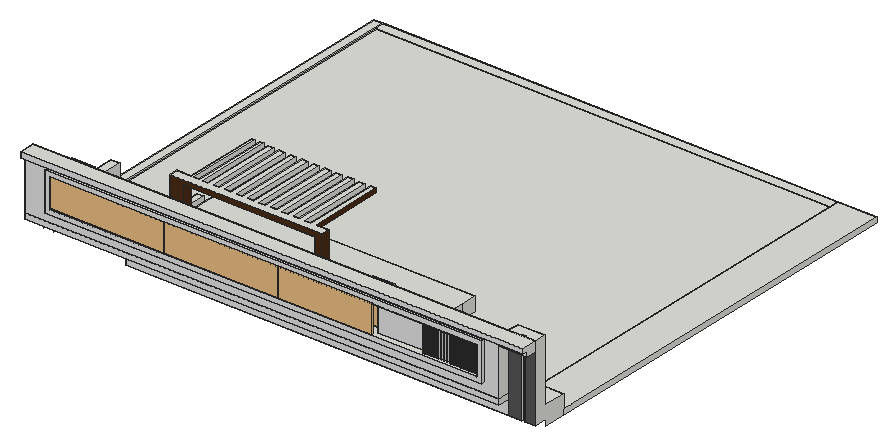
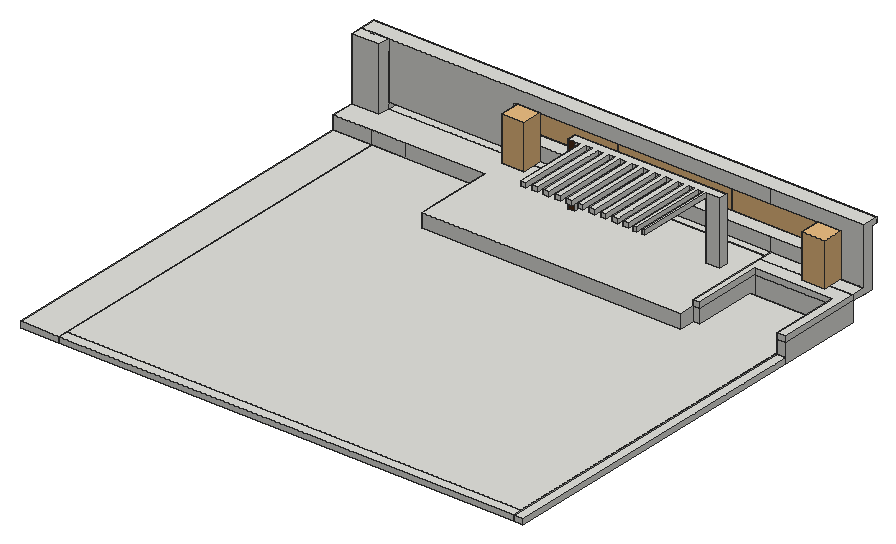
# SketchUp Ruby script. Lengths in inches.
U = 1.inch
M = Sketchup.active_model
def pt(a) = Geom::Point3d.new(a.map { |v| v * U })
def face(e, loops, mat)
  f = e.add_face(loops[0].map { |a| pt(a) })
  loops[1..].each { |l| e.add_face(l.map { |a| pt(a) }).erase! }
  f.material = f.back_material = mat if mat
  f
end
# faces: each face lists its corners as indices into pts; further lists are holes
def faces(e, pts, list, mat = nil) = list.each { |f| face(e, (f[0].is_a?(Array) ? f : [f]).map { |l| l.map { |i| pts[i] } }, mat) }
# xy, xz, yz: faces in a plane at the given z, y or x. An outline is a flat list of corners, or four numbers for a rectangle; further outlines are holes
def ring(l) = l.size == 4 ? [[l[0], l[1]], [l[2], l[1]], [l[2], l[3]], [l[0], l[3]]] : l.each_slice(2).to_a
def flat(e, list, mat, &to3) = list.each { |f| face(e, (f[0].is_a?(Array) ? f : [f]).map { |l| ring(l).map { |u, v| to3.(u, v) } }, mat) }
def xy(e, z, list, mat = nil) = flat(e, list, mat) { |x, y| [x, y, z] }
def xz(e, y, list, mat = nil) = flat(e, list, mat) { |x, z| [x, y, z] }
def yz(e, x, list, mat = nil) = flat(e, list, mat) { |y, z| [x, y, z] }
def lines(e, pts, list) = list.each { |a, b| e.add_line(pt(pts[a]), pt(pts[b])) }
# prism: a flat outline (further loops are holes) pulled along v
def prism(e, loops, v, mat = nil)
  f = face(e, loops, mat); d = Geom::Vector3d.new(v.map { |x| x * U })
  f.pushpull(f.normal.samedirection?(d) ? d.length : -d.length)
end
def box(e, o, s, mat = nil) = prism(e, [[o, [o[0] + s[0], o[1], o[2]], [o[0] + s[0], o[1] + s[1], o[2]], [o[0], o[1] + s[1], o[2]]]], [0, 0, s[2]], mat)
def at(x, y, z, deg = 0) = Geom::Transformation.translation(pt([x, y, z])) * Geom::Transformation.rotation(ORIGIN, Z_AXIS, deg.degrees)
def axes(o, x, y, z) = Geom::Transformation.new([*x, 0, *y, 0, *z, 0, *pt(o).to_a, 1])
def part(name) = M.definitions.add(name)
# library, detail: a bought-in or finely detailed component or shape, given as its bounding box
def library(name, o, s) = part(name).tap { |d| box(d.entities, o, s) }
def detail(e, o, s) = box(e.add_group.entities, o, s)
def put(e, d, t, mat = nil) = e.add_instance(d, t).tap { |i| i.material = mat if mat }
def group(e, t, mat = nil) = e.add_group.tap { |g| g.transformation = t; g.material = mat if mat }.entities
root = M.entities
M.materials.add("[Color M01]").color = [226, 226, 226]
M.materials.add("[Color M06]").color = [86, 86, 86]
M.materials.add("[Wood Veneer 01]").color = [76, 44, 23]
c1 = library("SPOT",[0,0,1.68],[5.4375,5.4375,6.28])
c2 = library("Yukka",[-2.74,-1.93,0],[38.67,34.64,74.8125])
c3 = part("glass-railing")
detail(c3.entities,[0,0,0],[1.26,75.59,33.1875])
xy(root,510,[[303.12,279.2,303.12,683.75,784.56,683.75,784.56,279.2,665.11,279.2,665.11,362.65,390.34,362.65,390.34,345.71,383.72,345.71,383.72,279.2],[383.72,279.2,390.34,345.71],[390.34,279.2,665.11,362.65],[784.56,279.2,825.43,694.43],[292.06,345.71,301.28,694.43],
  [301.28,683.75,784.56,694.43]])
xy(root,515.875,[[657.09,242.18,657.09,263.24,751.93,263.24,751.93,256.61,754.62,256.61,754.62,263.24,761.98,263.24,761.98,256.61,784.56,256.61,784.56,242.18],[784.56,242.18,784.56,256.61,811.07,256.61,811.07,258.49,814.72,258.49,814.72,256.61,825.43,256.61,825.43,242.18,813.93,242.18,813.93,244.11,810.6,244.11,810.6,242.18]])
xy(root,515.875,[[[390.34,242.18,657.09,345.71],[511.65,248.63,512.53,248.63,512.53,249.32,515.36,249.32,515.36,250.63,516,250.63,516,249.32,518.83,249.32,518.83,250.63,519.47,250.63,519.47,249.32,522.3,249.32,522.3,250.63,522.9375,250.63,522.9375,249.32,525.77,249.32,525.77,250.63,526.41,250.63,526.41,249.32,529.24,249.32,529.24,250.63,529.78,250.63,529.78,248.63,530.65,248.63,530.65,269.63,511.65,269.63],[595.53,289.875,596.83,289.96,598.07,290.37,599.16,291.09,600.02,292.07,600.61,293.24,600.87,294.52,600.79,295.82,600.37,297.06,599.65,298.14,598.67,299.01,597.51,299.59,596.23,299.85,594.92,299.77,593.6875,299.36,592.6,298.64,591.73,297.66,591.15,296.49,590.89,295.21,590.97,293.91,591.39,292.67,592.11,291.58,593.08,290.72,594.25,290.14],[447.91,289.875,449.21,289.96,450.45,290.37,451.53,291.09,452.4,292.07,452.98,293.24,453.24,294.52,453.16,295.82,452.75,297.06,452.03,298.14,451.05,299.01,449.88,299.59,448.6,299.85,447.3,299.77,446.0625,299.36,444.97,298.64,444.11,297.66,443.53,296.49,443.27,295.21,443.35,293.91,443.76,292.67,444.48,291.58,445.46,290.72,446.625,290.14]]],"[Wood Veneer 01]")
xy(root,516,[[303.12,279.2,784.56,683.75],[784.56,279.2,825.43,694.43],[292.06,345.71,301.28,694.43],[301.28,683.75,784.56,694.43]])
xy(root,516.9375,[[595.53,289.875,594.25,290.14,593.08,290.72,592.11,291.58,591.39,292.67,590.97,293.91,590.89,295.21,591.15,296.49,591.73,297.66,592.6,298.64,593.6875,299.36,594.92,299.77,596.23,299.85,597.51,299.59,598.67,299.01,599.65,298.14,600.37,297.06,600.79,295.82,600.87,294.52,600.61,293.24,600.02,292.07,599.16,291.09,598.07,290.37,596.83,289.96]])
xy(root,517.375,[[447.91,289.875,446.625,290.14,445.46,290.72,444.48,291.58,443.76,292.67,443.35,293.91,443.27,295.21,443.53,296.49,444.11,297.66,444.97,298.64,446.0625,299.36,447.3,299.77,448.6,299.85,449.88,299.59,451.05,299.01,452.03,298.14,452.75,297.06,453.16,295.82,453.24,294.52,452.98,293.24,452.4,292.07,451.53,291.09,450.45,290.37,449.21,289.96]])
xy(root,519.6875,[[302.78,256.61,380.53,263.24]])
xy(root,530.25,[[292.06,231.11,390.34,242.18],[390.34,231.11,795.77,242.18],[[390.34,242.18,795.77,242.18,797.0625,254.92,825.43,254.92,825.43,279.2,665.11,279.2,665.11,362.65,390.34,362.65],[413.19,272.63,428.05,281.82],[567.24,272.63,573.99,281.82]]])
xy(root,536.3125,[[292.06,231.11,795.77,242.18],[292.06,242.18,390.34,256.61],[292.06,256.61,390.34,256.61,390.34,345.71,383.72,345.71,383.72,272.46,301.28,272.46,301.28,345.71,292.06,345.71]])
xy(root,546.15,[[316.49,227.68,779.86,231.11]])
xy(root,550.91,[[321.25,227.68,775.1,227.68,775.1,232.24,773.26,232.24,773.26,234.93,771.98,234.93,771.98,232.24,770.13,232.24,770.13,234.93,768.85,234.93,768.85,232.24,767.01,232.24,767.01,234.93,765.73,234.93,765.73,232.24,763.88,232.24,763.88,234.93,762.6,234.93,762.6,232.24,760.76,232.24,760.76,234.93,759.48,234.93,759.48,232.24,757.63,232.24,757.63,234.93,756.35,234.93,756.35,232.24,754.51,232.24,754.51,234.93,753.23,234.93,753.23,232.24,751.38,232.24,751.38,234.93,750.1,234.93,750.1,232.24,748.26,232.24,748.26,234.93,746.98,234.93,746.98,232.24,745.13,232.24,745.13,234.93,743.85,234.93,743.85,232.24,742.01,232.24,742.01,234.93,740.73,234.93,740.73,232.24,738.88,232.24,738.88,234.93,737.6,234.93,737.6,232.24,735.76,232.24,735.76,234.93,734.48,234.93,734.48,232.24,732.63,232.24,732.63,234.93,731.35,234.93,731.35,232.24,729.51,232.24,729.51,234.93,728.23,234.93,728.23,232.24,726.38,232.24,726.38,234.93,725.1,234.93,725.1,232.24,723.26,232.24,723.26,234.93,721.98,234.93,721.98,232.24,720.13,232.24,720.13,234.93,719.1,234.93,719.1,232.24,717.26,232.24,717.26,234.93,716.23,234.93,716.23,231.3,714.38,231.3,714.38,234.93,663.67,234.93,663.67,242.18,321.25,242.18],[714.38,231.3,716.23,233.99],[717.26,232.24,719.1,234.93],[720.13,232.24,721.98,234.93],[723.26,232.24,725.1,234.93],
  [726.38,232.24,728.23,234.93],[729.51,232.24,731.35,234.93],[732.63,232.24,734.48,234.93],[735.76,232.24,737.6,234.93],[738.88,232.24,740.73,234.93],
  [742.01,232.24,743.85,234.93],[745.13,232.24,746.98,234.93],[748.26,232.24,750.1,234.93],[751.38,232.24,753.23,234.93],[754.51,232.24,756.35,234.93],
  [757.63,232.24,759.48,234.93],[760.76,232.24,762.6,234.93],[763.88,232.24,765.73,234.93],[767.01,232.24,768.85,234.93],[770.13,232.24,771.98,234.18],
  [773.26,232.24,775.1,232.99],[773.26,232.99,775.1,234.93],[714.38,233.99,716.23,234.3],[770.13,234.18,771.98,234.61],[770.13,234.61,771.98,234.93]])
xy(root,582.02,[[321.25,227.68,321.25,242.18,663.67,242.18,663.67,234.93,714.38,234.93,714.38,231.3,716.23,231.3,716.23,234.93,717.26,234.93,717.26,232.24,719.1,232.24,719.1,234.93,720.13,234.93,720.13,232.24,721.98,232.24,721.98,234.93,723.26,234.93,723.26,232.24,725.1,232.24,725.1,234.93,726.38,234.93,726.38,232.24,728.23,232.24,728.23,234.93,729.51,234.93,729.51,232.24,731.35,232.24,731.35,234.93,732.63,234.93,732.63,232.24,734.48,232.24,734.48,234.93,735.76,234.93,735.76,232.24,737.6,232.24,737.6,234.93,738.88,234.93,738.88,232.24,740.73,232.24,740.73,234.93,742.01,234.93,742.01,232.24,743.85,232.24,743.85,234.93,745.13,234.93,745.13,232.24,746.98,232.24,746.98,234.93,748.26,234.93,748.26,232.24,750.1,232.24,750.1,234.93,751.38,234.93,751.38,232.24,753.23,232.24,753.23,234.93,754.51,234.93,754.51,232.24,756.35,232.24,756.35,234.93,757.63,234.93,757.63,232.24,759.48,232.24,759.48,234.93,760.76,234.93,760.76,232.24,762.6,232.24,762.6,234.93,763.88,234.93,763.88,232.24,765.73,232.24,765.73,234.93,767.01,234.93,767.01,232.24,768.85,232.24,768.85,234.93,770.13,234.93,770.13,232.24,771.98,232.24,771.98,234.93,773.26,234.93,773.26,232.24,775.1,232.24,775.1,227.68],[714.38,231.3,716.23,233.99],[717.26,232.24,719.1,234.93],[720.13,232.24,721.98,234.93],[723.26,232.24,725.1,234.93],
  [726.38,232.24,728.23,234.93],[729.51,232.24,731.35,234.93],[732.63,232.24,734.48,234.93],[735.76,232.24,737.6,234.93],[738.88,232.24,740.73,234.93],
  [742.01,232.24,743.85,234.93],[745.13,232.24,746.98,234.93],[748.26,232.24,750.1,234.93],[751.38,232.24,753.23,234.93],[754.51,232.24,756.35,234.93],
  [757.63,232.24,759.48,234.93],[760.76,232.24,762.6,234.93],[763.88,232.24,765.73,234.93],[767.01,232.24,768.85,234.93],[770.13,232.24,771.98,234.18],
  [773.26,232.24,775.1,232.99],[773.26,232.99,775.1,234.93],[714.38,233.99,716.23,234.3],[770.13,234.18,771.98,234.61],[770.13,234.61,771.98,234.93]])
xy(root,586.3,[[795.77,231.11,825.43,242.18]])
xy(root,586.78,[[316.49,227.68,779.86,231.11]])
xy(root,591.86,[[428.05,272.63,428.05,362.65,431.14,362.65,431.14,281.82,436.78,281.82,436.78,362.65,440.71,362.65,440.71,281.82,445.99,281.82,445.99,361.33,452.05,361.33,452.05,281.82,458.11,281.82,458.11,361.33,464.18,361.33,464.18,281.82,470.24,281.82,470.24,361.33,476.3,361.33,476.3,281.82,482.36,281.82,482.36,361.33,488.43,361.33,488.43,281.82,494.49,281.82,494.49,361.33,500.55,361.33,500.55,281.82,506.61,281.82,506.61,361.33,512.68,361.33,512.68,281.82,518.74,281.82,518.74,361.33,524.8,361.33,524.8,281.82,530.86,281.82,530.86,361.33,536.93,361.33,536.93,281.82,542.99,281.82,542.99,361.33,549.05,361.33,549.05,281.82,555.11,281.82,555.11,361.33,561.18,361.33,561.18,281.82,567.24,281.82,567.24,272.63]],"[Wood Veneer 01]")
xy(root,596.625,[[292.06,225.49,825.43,242.18],[795.77,242.18,810.6,242.18,810.6,244.11,813.93,244.11,813.93,242.18,825.43,242.18,825.43,254.92,797.0625,254.92],[413.19,272.63,573.99,272.63,573.99,281.82,561.18,281.82,561.18,361.33,555.11,361.33,555.11,281.82,549.05,281.82,549.05,361.33,542.99,361.33,542.99,281.82,536.93,281.82,536.93,361.33,530.86,361.33,530.86,281.82,524.8,281.82,524.8,361.33,518.74,361.33,518.74,281.82,512.68,281.82,512.68,361.33,506.61,361.33,506.61,281.82,500.55,281.82,500.55,361.33,494.49,361.33,494.49,281.82,488.43,281.82,488.43,361.33,482.36,361.33,482.36,281.82,476.3,281.82,476.3,361.33,470.24,361.33,470.24,281.82,464.18,281.82,464.18,361.33,458.11,361.33,458.11,281.82,452.05,281.82,452.05,361.33,445.99,361.33,445.99,281.82,440.71,281.82,440.71,362.65,436.78,362.65,436.78,281.82,431.14,281.82,431.14,362.65,428.05,362.65,428.05,281.82,413.19,281.82]])
xz(root,225.49,[[292.06,590.76,825.43,591.46,825.43,596.625,292.06,596.625]],"[Color M01]")
xz(root,227.68,[[[316.49,546.15,779.86,586.78],[321.25,550.91,775.1,582.02]]],"[Color M01]")
xz(root,231.11,[[292.06,530.25,795.77,536.3125],[[292.06,536.3125,795.77,536.3125,795.77,586.3,825.43,586.3,825.43,591.46,292.06,590.76],[316.49,546.15,779.86,586.78]]],"[Color M01]")
xz(root,231.3,[[714.38,550.91,716.23,582.02]],"[Wood Veneer 01]")
xz(root,232.24,[[717.26,550.91,719.1,582.02],[720.13,550.91,721.98,582.02],[723.26,550.91,725.1,582.02],[726.38,550.91,728.23,582.02],[729.51,550.91,731.35,582.02],
  [732.63,550.91,734.48,582.02],[735.76,550.91,737.6,582.02],[738.88,550.91,740.73,582.02],[742.01,550.91,743.85,582.02],[745.13,550.91,746.98,582.02],
  [748.26,550.91,750.1,582.02],[751.38,550.91,753.23,582.02],[754.51,550.91,756.35,582.02],[757.63,550.91,759.48,582.02],[760.76,550.91,762.6,582.02],
  [763.88,550.91,765.73,582.02],[767.01,550.91,768.85,582.02],[770.13,550.91,771.98,582.02],[773.26,550.91,775.1,582.02]],"[Wood Veneer 01]")
xz(root,232.99,[[773.26,550.91,775.1,582.02]])
xz(root,233.99,[[714.38,550.91,716.23,582.02]])
xz(root,234.18,[[770.13,550.91,771.98,582.02]])
xz(root,234.3,[[714.38,550.91,716.23,582.02]])
xz(root,234.61,[[770.13,550.91,771.98,582.02]])
xz(root,234.93,[[716.23,550.91,717.26,582.02],[717.26,550.91,719.1,582.02],[719.1,550.91,720.13,582.02],[720.13,550.91,721.98,582.02],[721.98,550.91,723.26,582.02],
  [723.26,550.91,725.1,582.02],[725.1,550.91,726.38,582.02],[726.38,550.91,728.23,582.02],[728.23,550.91,729.51,582.02],[729.51,550.91,731.35,582.02],
  [731.35,550.91,732.63,582.02],[732.63,550.91,734.48,582.02],[734.48,550.91,735.76,582.02],[735.76,550.91,737.6,582.02],[737.6,550.91,738.88,582.02],
  [738.88,550.91,740.73,582.02],[740.73,550.91,742.01,582.02],[742.01,550.91,743.85,582.02],[743.85,550.91,745.13,582.02],[745.13,550.91,746.98,582.02],
  [746.98,550.91,748.26,582.02],[748.26,550.91,750.1,582.02],[750.1,550.91,751.38,582.02],[751.38,550.91,753.23,582.02],[753.23,550.91,754.51,582.02],
  [754.51,550.91,756.35,582.02],[756.35,550.91,757.63,582.02],[757.63,550.91,759.48,582.02],[759.48,550.91,760.76,582.02],[760.76,550.91,762.6,582.02],
  [762.6,550.91,763.88,582.02],[763.88,550.91,765.73,582.02],[765.73,550.91,767.01,582.02],[767.01,550.91,768.85,582.02],[768.85,550.91,770.13,582.02],
  [770.13,550.91,771.98,582.02],[771.98,550.91,773.26,582.02],[773.26,550.91,775.1,582.02]])
xz(root,234.93,[[663.67,550.91,714.38,582.02]],"[Color M01]")
xz(root,242.18,[[292.06,530.25,390.34,536.3125],[292.06,536.3125,292.06,596.625,390.34,596.625,390.34,582.02,321.25,582.02,321.25,550.91,390.34,550.91,390.34,536.3125],[390.34,536.3125,390.34,550.91,663.67,550.91,663.67,582.02,390.34,582.02,390.34,596.625,795.77,596.625,795.77,536.3125],[795.77,586.3,810.6,596.625],[810.6,586.3,813.93,596.625],
  [813.93,586.3,825.43,596.625]])
xz(root,242.18,[[390.34,515.875,795.77,530.25]],"[Color M01]")
xz(root,242.18,[[795.77,515.875,810.6,586.3],[813.93,515.875,825.43,586.3]],"[Color M06]")
xz(root,254.92,[[797.0625,530.25,825.43,596.625]])
xz(root,256.61,[[292.06,530.25,390.34,536.3125]])
xz(root,272.46,[[301.28,510,383.72,530.25],[301.28,530.25,383.72,536.3125]])
xz(root,272.63,[[413.19,530.25,428.05,530.25,428.05,591.86,567.24,591.86,567.24,530.25,573.99,530.25,573.99,596.625,413.19,596.625]],"[Wood Veneer 01]")
xz(root,279.2,[[303.12,510,665.11,516],[665.11,510,749.59,516],[749.59,510,784.56,516],[784.56,510,825.43,516],[665.11,516,749.59,530.25],
  [749.59,516,784.56,530.25],[784.56,516,825.43,530.25]])
xz(root,281.82,[[413.19,530.25,428.05,596.625],[431.14,591.86,436.78,596.625],[440.71,591.86,445.99,596.625],[452.05,591.86,458.11,596.625],[464.18,591.86,470.24,596.625],
  [476.3,591.86,482.36,596.625],[488.43,591.86,494.49,596.625],[500.55,591.86,506.61,596.625],[512.68,591.86,518.74,596.625],[524.8,591.86,530.86,596.625],
  [536.93,591.86,542.99,596.625],[549.05,591.86,555.11,596.625],[561.18,591.86,567.24,596.625]])
xz(root,281.82,[[567.24,530.25,573.99,596.625]],"[Wood Veneer 01]")
xz(root,345.71,[[292.06,510,301.28,516],[383.72,510,390.34,530.25],[292.06,516,301.28,530.25],[292.06,530.25,301.28,536.3125],[383.72,530.25,390.34,536.3125]])
xz(root,361.33,[[445.99,591.86,452.05,596.625],[458.11,591.86,464.18,596.625],[470.24,591.86,476.3,596.625],[482.36,591.86,488.43,596.625],[494.49,591.86,500.55,596.625],
  [506.61,591.86,512.68,596.625],[518.74,591.86,524.8,596.625],[530.86,591.86,536.93,596.625],[542.99,591.86,549.05,596.625],[555.11,591.86,561.18,596.625]])
xz(root,362.65,[[390.34,510,665.11,530.25],[428.05,591.86,431.14,596.625],[436.78,591.86,440.71,596.625]])
xz(root,683.75,[[301.28,510,303.12,516],[303.12,510,784.56,516]])
xz(root,694.43,[[292.06,510,301.28,516],[301.28,510,784.56,516],[784.56,510,825.43,516]])
yz(root,292.06,[[256.61,510,345.71,530.25],[345.71,510,694.43,516],[231.11,530.25,231.11,590.76,225.49,590.76,225.49,596.625,242.18,596.625,242.18,536.3125,256.61,536.3125,256.61,530.25],[256.61,530.25,345.71,536.3125]])
yz(root,301.28,[[272.46,510,345.71,536.3125],[345.71,510,683.75,516],[683.75,510,694.43,516]])
yz(root,302.78,[[256.61,510,263.24,519.6875]])
yz(root,303.12,[[279.2,510,683.75,516]])
yz(root,316.49,[[227.68,546.15,231.11,586.78]])
yz(root,321.25,[[227.68,550.91,242.18,582.02]])
yz(root,380.53,[[256.61,510,263.24,519.6875]])
yz(root,383.72,[[272.46,510,345.71,530.25],[272.46,530.25,345.71,536.3125]])
yz(root,390.34,[[256.61,510,272.46,515.875],[272.46,510,345.71,515.875],[345.71,510,362.65,530.25],[242.18,515.875,256.61,530.25],[256.61,515.875,272.46,530.25],
  [272.46,515.875,345.71,530.25],[242.18,530.25,256.61,536.3125],[256.61,530.25,272.46,536.3125],[272.46,530.25,345.71,536.3125]])
yz(root,413.19,[[272.63,530.25,281.82,596.625]])
yz(root,428.05,[[281.82,591.86,362.65,596.625]])
yz(root,428.05,[[272.63,530.25,281.82,591.86]],"[Wood Veneer 01]")
yz(root,431.14,[[281.82,591.86,362.65,596.625]])
yz(root,436.78,[[281.82,591.86,362.65,596.625]])
yz(root,440.71,[[281.82,591.86,362.65,596.625]])
yz(root,445.99,[[281.82,591.86,361.33,596.625]])
yz(root,452.05,[[281.82,591.86,361.33,596.625]])
yz(root,458.11,[[281.82,591.86,361.33,596.625]])
yz(root,464.18,[[281.82,591.86,361.33,596.625]])
yz(root,470.24,[[281.82,591.86,361.33,596.625]])
yz(root,476.3,[[281.82,591.86,361.33,596.625]])
yz(root,482.36,[[281.82,591.86,361.33,596.625]])
yz(root,488.43,[[281.82,591.86,361.33,596.625]])
yz(root,494.49,[[281.82,591.86,361.33,596.625]])
yz(root,500.55,[[281.82,591.86,361.33,596.625]])
yz(root,506.61,[[281.82,591.86,361.33,596.625]])
yz(root,512.68,[[281.82,591.86,361.33,596.625]])
yz(root,518.74,[[281.82,591.86,361.33,596.625]])
yz(root,524.8,[[281.82,591.86,361.33,596.625]])
yz(root,530.86,[[281.82,591.86,361.33,596.625]])
yz(root,536.93,[[281.82,591.86,361.33,596.625]])
yz(root,542.99,[[281.82,591.86,361.33,596.625]])
yz(root,549.05,[[281.82,591.86,361.33,596.625]])
yz(root,555.11,[[281.82,591.86,361.33,596.625]])
yz(root,561.18,[[281.82,591.86,361.33,596.625]],"[Wood Veneer 01]")
yz(root,567.24,[[272.63,530.25,281.82,591.86]])
yz(root,573.99,[[272.63,530.25,281.82,596.625]],"[Wood Veneer 01]")
yz(root,663.67,[[234.93,550.91,242.18,582.02]])
yz(root,665.11,[[279.2,510,345.71,530.25],[345.71,510,362.65,530.25]])
yz(root,714.38,[[231.3,550.91,233.99,582.02],[233.99,550.91,234.3,582.02],[234.3,550.91,234.93,582.02]])
yz(root,716.23,[[231.3,550.91,233.99,582.02],[233.99,550.91,234.3,582.02],[234.3,550.91,234.93,582.02]])
yz(root,717.26,[[232.24,550.91,234.93,582.02]])
yz(root,719.1,[[232.24,550.91,234.93,582.02]])
yz(root,720.13,[[232.24,550.91,234.93,582.02]])
yz(root,721.98,[[232.24,550.91,234.93,582.02]])
yz(root,723.26,[[232.24,550.91,234.93,582.02]])
yz(root,725.1,[[232.24,550.91,234.93,582.02]])
yz(root,726.38,[[232.24,550.91,234.93,582.02]])
yz(root,728.23,[[232.24,550.91,234.93,582.02]])
yz(root,729.51,[[232.24,550.91,234.93,582.02]])
yz(root,731.35,[[232.24,550.91,234.93,582.02]])
yz(root,732.63,[[232.24,550.91,234.93,582.02]])
yz(root,734.48,[[232.24,550.91,234.93,582.02]])
yz(root,735.76,[[232.24,550.91,234.93,582.02]])
yz(root,737.6,[[232.24,550.91,234.93,582.02]])
yz(root,738.88,[[232.24,550.91,234.93,582.02]])
yz(root,740.73,[[232.24,550.91,234.93,582.02]])
yz(root,742.01,[[232.24,550.91,234.93,582.02]])
yz(root,743.85,[[232.24,550.91,234.93,582.02]])
yz(root,745.13,[[232.24,550.91,234.93,582.02]])
yz(root,746.98,[[232.24,550.91,234.93,582.02]])
yz(root,748.26,[[232.24,550.91,234.93,582.02]])
yz(root,750.1,[[232.24,550.91,234.93,582.02]])
yz(root,751.38,[[232.24,550.91,234.93,582.02]])
yz(root,753.23,[[232.24,550.91,234.93,582.02]])
yz(root,754.51,[[232.24,550.91,234.93,582.02]])
yz(root,756.35,[[232.24,550.91,234.93,582.02]])
yz(root,757.63,[[232.24,550.91,234.93,582.02]])
yz(root,759.48,[[232.24,550.91,234.93,582.02]])
yz(root,760.76,[[232.24,550.91,234.93,582.02]])
yz(root,762.6,[[232.24,550.91,234.93,582.02]])
yz(root,763.88,[[232.24,550.91,234.93,582.02]])
yz(root,765.73,[[232.24,550.91,234.93,582.02]])
yz(root,767.01,[[232.24,550.91,234.93,582.02]])
yz(root,768.85,[[232.24,550.91,234.93,582.02]])
yz(root,770.13,[[232.24,550.91,234.18,582.02],[234.18,550.91,234.61,582.02],[234.61,550.91,234.93,582.02]])
yz(root,771.98,[[232.24,550.91,234.18,582.02],[234.18,550.91,234.61,582.02],[234.61,550.91,234.93,582.02]])
yz(root,773.26,[[232.24,550.91,232.99,582.02],[232.99,550.91,234.93,582.02]])
yz(root,775.1,[[227.68,550.91,232.24,582.02],[232.24,550.91,232.99,582.02],[232.99,550.91,234.93,582.02]])
yz(root,779.86,[[227.68,546.15,231.11,586.78]])
yz(root,784.56,[[279.2,510,683.75,516],[683.75,510,694.43,516]])
yz(root,795.77,[[231.11,530.25,242.18,536.3125],[231.11,536.3125,242.18,586.3]])
yz(root,810.6,[[242.18,515.875,244.11,596.625]])
yz(root,813.93,[[242.18,515.875,244.11,596.625]])
yz(root,825.43,[[256.61,510,279.2,510,279.2,530.25,254.92,530.25,254.92,596.625,242.18,596.625,242.18,515.875,256.61,515.875],[279.2,510,694.43,516],[231.11,586.3,242.18,586.3,242.18,596.625,225.49,596.625,225.49,591.46,231.11,591.46]])
p = [[447.91,289.875,515.875],[446.625,290.14,515.875],[446.625,290.14,517.375],[447.91,289.875,517.375],[449.21,289.96,515.875],[449.21,289.96,517.375],
  [595.53,289.875,515.875],[594.25,290.14,515.875],[594.25,290.14,516.9375],[595.53,289.875,516.9375],[596.83,289.96,515.875],[596.83,289.96,516.9375],
  [450.45,290.37,515.875],[450.45,290.37,517.375],[598.07,290.37,515.875],[598.07,290.37,516.9375],[445.46,290.72,515.875],[445.46,290.72,517.375],
  [593.08,290.72,515.875],[593.08,290.72,516.9375],[451.53,291.09,515.875],[451.53,291.09,517.375],[599.16,291.09,515.875],[599.16,291.09,516.9375],
  [444.48,291.58,515.875],[444.48,291.58,517.375],[592.11,291.58,515.875],[592.11,291.58,516.9375],[452.4,292.07,515.875],[452.4,292.07,517.375],
  [600.02,292.07,515.875],[600.02,292.07,516.9375],[443.76,292.67,515.875],[443.76,292.67,517.375],[591.39,292.67,515.875],[591.39,292.67,516.9375],
  [452.98,293.24,515.875],[452.98,293.24,517.375],[600.61,293.24,515.875],[600.61,293.24,516.9375],[443.35,293.91,515.875],[443.35,293.91,517.375],
  [590.97,293.91,515.875],[590.97,293.91,516.9375],[453.24,294.52,515.875],[453.24,294.52,517.375],[600.87,294.52,515.875],[600.87,294.52,516.9375],
  [443.27,295.21,515.875],[443.27,295.21,517.375],[590.89,295.21,515.875],[590.89,295.21,516.9375],[453.16,295.82,515.875],[453.16,295.82,517.375],
  [600.79,295.82,515.875],[600.79,295.82,516.9375],[443.53,296.49,515.875],[443.53,296.49,517.375],[591.15,296.49,515.875],[591.15,296.49,516.9375],
  [452.75,297.06,515.875],[452.75,297.06,517.375],[600.37,297.06,515.875],[600.37,297.06,516.9375],[444.11,297.66,515.875],[444.11,297.66,517.375],
  [591.73,297.66,515.875],[591.73,297.66,516.9375],[452.03,298.14,515.875],[452.03,298.14,517.375],[599.65,298.14,515.875],[599.65,298.14,516.9375],
  [444.97,298.64,515.875],[444.97,298.64,517.375],[592.6,298.64,515.875],[592.6,298.64,516.9375],[451.05,299.01,515.875],[451.05,299.01,517.375],
  [598.67,299.01,515.875],[598.67,299.01,516.9375],[446.0625,299.36,515.875],[446.0625,299.36,517.375],[593.6875,299.36,515.875],[593.6875,299.36,516.9375],
  [449.88,299.59,515.875],[449.88,299.59,517.375],[597.51,299.59,515.875],[597.51,299.59,516.9375],[447.3,299.77,515.875],[447.3,299.77,517.375],
  [594.92,299.77,515.875],[594.92,299.77,516.9375],[448.6,299.85,515.875],[448.6,299.85,517.375],[596.23,299.85,515.875],[596.23,299.85,516.9375],
  [797.0625,254.92,530.25],[795.77,242.18,530.25],[795.77,242.18,536.3125],[795.77,242.18,586.3],[795.77,242.18,596.625],[797.0625,254.92,596.625],
  [292.06,231.11,590.76],[825.43,231.11,591.46],[825.43,225.49,591.46],[292.06,225.49,590.76],[784.56,263.24,510],[784.56,279.2,510]]
faces(root,p,[[0,1,2,3],[4,0,3,5],[6,7,8,9],[10,6,9,11],[12,4,5,13],[14,10,11,15],[1,16,17,2],[7,18,19,8],
  [20,12,13,21],[22,14,15,23],[16,24,25,17],[18,26,27,19],[28,20,21,29],[30,22,23,31],[24,32,33,25],[26,34,35,27],
  [36,28,29,37],[38,30,31,39],[32,40,41,33],[34,42,43,35],[44,36,37,45],[46,38,39,47],[40,48,49,41],[42,50,51,43],
  [52,44,45,53],[54,46,47,55],[48,56,57,49],[50,58,59,51],[60,52,53,61],[62,54,55,63],[56,64,65,57],[58,66,67,59],
  [68,60,61,69],[70,62,63,71],[64,72,73,65],[66,74,75,67],[76,68,69,77],[78,70,71,79],[72,80,81,73],[74,82,83,75],
  [84,76,77,85],[86,78,79,87],[80,88,89,81],[82,90,91,83],[92,84,85,93],[94,86,87,95],[88,92,93,89],[90,94,95,91],
  [96,97,98,99,100,101],[102,103,104,105]])
lines(root,p,[[106,107]])
put(root,c1,at(593.24,293.57,508.89))
put(root,c2,axes([318.23,243.54,536.3125],[0.62,0,0],[0,0.62,0],[0,0,0.62]))
put(root,c2,axes([637.04,243.54,536.3125],[0.62,0,0],[0,0.62,0],[0,0,0.62]))
put(root,c3,axes([563.61,229.3,552.18],[0,-1.29,0],[1.32371,0,0],[0,0,0.89905]))
put(root,c3,axes([321.25,229.3,552.18],[0,-1.29,0],[1.60489,0,0],[0,0,0.89905]))
put(root,c3,axes([442.43,229.3,552.18],[0,-1.29,0],[1.60489,0,0],[0,0,0.89905]))
